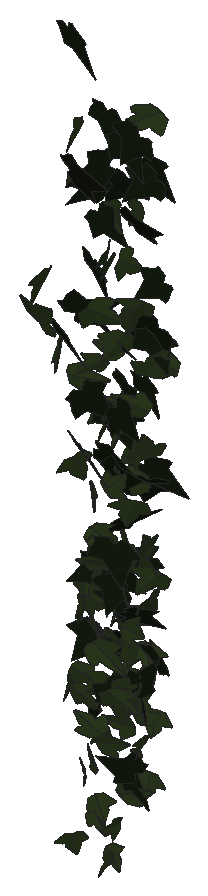
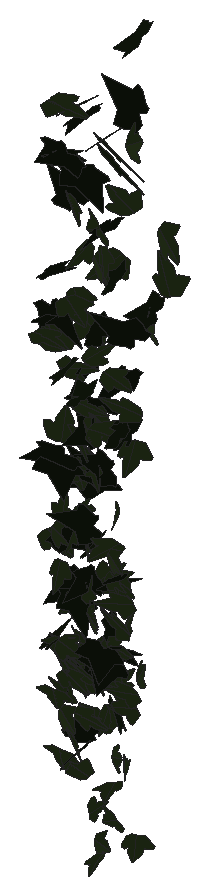
# SketchUp Ruby script. Lengths in inches.
U = 1.inch
M = Sketchup.active_model
def pt(a) = Geom::Point3d.new(a.map { |v| v * U })
def face(e, loops, mat)
  f = e.add_face(loops[0].map { |a| pt(a) })
  loops[1..].each { |l| e.add_face(l.map { |a| pt(a) }).erase! }
  f.material = f.back_material = mat if mat
  f
end
# faces: each face lists its corners as indices into pts; further lists are holes
def faces(e, pts, list, mat = nil) = list.each { |f| face(e, (f[0].is_a?(Array) ? f : [f]).map { |l| l.map { |i| pts[i] } }, mat) }
# xy, xz, yz: faces in a plane at the given z, y or x. An outline is a flat list of corners, or four numbers for a rectangle; further outlines are holes
def ring(l) = l.size == 4 ? [[l[0], l[1]], [l[2], l[1]], [l[2], l[3]], [l[0], l[3]]] : l.each_slice(2).to_a
def flat(e, list, mat, &to3) = list.each { |f| face(e, (f[0].is_a?(Array) ? f : [f]).map { |l| ring(l).map { |u, v| to3.(u, v) } }, mat) }
def xy(e, z, list, mat = nil) = flat(e, list, mat) { |x, y| [x, y, z] }
def xz(e, y, list, mat = nil) = flat(e, list, mat) { |x, z| [x, y, z] }
def yz(e, x, list, mat = nil) = flat(e, list, mat) { |y, z| [x, y, z] }
def lines(e, pts, list) = list.each { |a, b| e.add_line(pt(pts[a]), pt(pts[b])) }
# prism: a flat outline (further loops are holes) pulled along v
def prism(e, loops, v, mat = nil)
  f = face(e, loops, mat); d = Geom::Vector3d.new(v.map { |x| x * U })
  f.pushpull(f.normal.samedirection?(d) ? d.length : -d.length)
end
def box(e, o, s, mat = nil) = prism(e, [[o, [o[0] + s[0], o[1], o[2]], [o[0] + s[0], o[1] + s[1], o[2]], [o[0], o[1] + s[1], o[2]]]], [0, 0, s[2]], mat)
def at(x, y, z, deg = 0) = Geom::Transformation.translation(pt([x, y, z])) * Geom::Transformation.rotation(ORIGIN, Z_AXIS, deg.degrees)
def axes(o, x, y, z) = Geom::Transformation.new([*x, 0, *y, 0, *z, 0, *pt(o).to_a, 1])
def part(name) = M.definitions.add(name)
# library, detail: a bought-in or finely detailed component or shape, given as its bounding box
def library(name, o, s) = part(name).tap { |d| box(d.entities, o, s) }
def detail(e, o, s) = box(e.add_group.entities, o, s)
def put(e, d, t, mat = nil) = e.add_instance(d, t).tap { |i| i.material = mat if mat }
def group(e, t, mat = nil) = e.add_group.tap { |g| g.transformation = t; g.material = mat if mat }.entities
root = M.entities
M.materials.add("1026 AP 7946 SUNNY SIDE UP").color = [254, 231, 186]
M.materials.add("efeu1").color = [18, 25, 13]
M.materials.add("efeu2").color = [43, 57, 29]
c1 = part("ivyleaf_10")
p = [[0,0.5,-0.03],[-0.0625,2.02,-0.43],[-0.19,2.01,-0.46],[-0.54,1.05,-0.29],[-0.52,0.625,-0.18],[-0.83,0.76,-0.28],
  [-1.16,0.64,-0.33],[-1.15,0.33,-0.24],[-0.77,-0.39,0.02],[-0.3,-0.51,0.16],[0.04,-0.48,0.23],[-0.02,2.01,-0.4375],
  [-0.06,2.01,-0.43],[0.04,-0.49,0.23],[0.67,-0.49,0.14],[1.38,0.36,-0.2],[1.375,0.51,-0.24],[0.81,0.65,-0.19],
  [0.62,0.59,-0.15],[0.6,1.09,-0.28],[0.5,1.23,-0.31]]
faces(c1.entities,p,[[0,1,2,3,4,5,6,7,8,9,10],[11,12,0,13,14,15,16,17,18,19,20]],"efeu2")
c2 = part("ivyleaf_9")
p = [[1.54,2.16,1.25],[1.36,2.04,1.19],[-0.21,0.99,0.68],[-0.71,1.11,0.82],[-0.85,0.86,0.67],[-0.8,0.17,0.21],
  [-0.9,-0.01,0.1],[-0.67,-0.16,-0.02],[-0.08,-0.08,-0.05],[-0.03,-0.6,-0.4],[0.65,-0.88,-0.66],[0.83,-0.6,-0.49],
  [1.29,-0.42,-0.43],[1.8125,-0.07,-0.26],[1.21,0.44,0.15]]
faces(c2.entities,p,[[0,1,2,3,4,5,6,7,8,9,10,11,12,13,14]],"efeu1")
put(root,c1,axes([106.32,210.03,262.625],[0.08292,-0.31995,0.11678],[0.03412,-0.11315,-0.33471],[0.5336,0.05695,0.00326]),"1026 AP 7946 SUNNY SIDE UP")
put(root,c2,axes([107.03,210.0625,265.32],[0.36461,-0.08477,-0.26189],[0.41394,0.01257,0.24359],[-0.07483,-0.3435,0.07141]),"1026 AP 7946 SUNNY SIDE UP")
put(root,c1,axes([106.15,210.07,261.48],[-0.42812,0.06677,0.19799],[0.28105,-0.07357,0.28733],[0.15166,0.32482,0.02646]),"1026 AP 7946 SUNNY SIDE UP")
put(root,c1,axes([107.52,210.3125,254.02],[0.2513,0.07628,0.2158],[0.32134,0.05151,-0.18003],[-0.13844,0.25804,-0.02615]),"1026 AP 7946 SUNNY SIDE UP")
put(root,c1,axes([106.29,210.54,260.7],[0.12846,-0.09926,0.28623],[0.25636,-0.22579,-0.13354],[0.38765,0.18221,-0.00653]),"1026 AP 7946 SUNNY SIDE UP")
put(root,c2,axes([107.8,210.52,256.46],[-0.16884,-0.23575,-0.10816],[0.09206,0.08701,-0.26586],[0.39433,-0.12125,0.01575]),"1026 AP 7946 SUNNY SIDE UP")
put(root,c1,axes([107.26,210.54,251.91],[0.14816,0.17283,0.13537],[-0.1153,-0.10836,0.20187],[0.32033,-0.11894,0.01005]),"1026 AP 7946 SUNNY SIDE UP")
put(root,c2,axes([106.14,210.61,261.12],[0.282,-0.2341,0.08241],[0.05534,-0.07531,-0.30373],[0.38573,0.18195,-0.01667]),"1026 AP 7946 SUNNY SIDE UP")
put(root,c1,axes([107.27,210.46,261.93],[-0.17759,-0.15909,-0.25489],[0.26554,0.18076,-0.19882],[0.37724,-0.20212,0.01995]),"1026 AP 7946 SUNNY SIDE UP")
put(root,c1,axes([106.34,210.83,252.49],[0.01742,0.01744,0.23633],[0.18302,-0.19843,0.00859],[0.31187,0.11547,-0.01824]),"1026 AP 7946 SUNNY SIDE UP")
put(root,c2,axes([106.57,210.89,258.23],[0.2136,-0.22227,0.16698],[0.10655,-0.14961,-0.26866],[0.42044,0.15084,-0.01675]),"1026 AP 7946 SUNNY SIDE UP")
put(root,c1,axes([107.51,210.83,252.68],[-0.27027,-0.05091,-0.17004],[0.26003,0.01732,-0.18313],[0.0769,-0.23747,0.02163]),"1026 AP 7946 SUNNY SIDE UP")
put(root,c1,axes([107.79,211.07,255.99],[-0.07859,-0.04134,0.25897],[0.06328,-0.25447,-0.03633],[0.39593,0.03246,0.05721]),"1026 AP 7946 SUNNY SIDE UP")
put(root,c2,axes([107.63,210.81,259.52],[0.14484,-0.18388,-0.23359],[-0.18555,0.19282,-0.21033],[0.41847,0.14915,-0.01241]),"1026 AP 7946 SUNNY SIDE UP")
put(root,c1,axes([106.47,210.87,257.91],[-0.16445,-0.25388,-0.116],[0.10257,0.09292,-0.28132],[0.42355,-0.12108,0.02309]),"1026 AP 7946 SUNNY SIDE UP")
put(root,c2,axes([107.12,210.98,264.7],[-0.41527,0.1572,-0.06447],[0.06317,-0.05612,-0.31572],[-0.25899,-0.26576,0.02637]),"1026 AP 7946 SUNNY SIDE UP")
put(root,c2,axes([106.125,211.11,267.87],[0.23929,-0.28624,0.02162],[-0.00227,-0.02636,-0.33383],[0.45148,0.15158,-0.01314]),"1026 AP 7946 SUNNY SIDE UP")
put(root,c2,axes([106.69,210.88,259.59],[0.06429,-0.13201,-0.28736],[-0.10817,0.26962,-0.14065],[0.47194,0.07978,0.00691]),"1026 AP 7946 SUNNY SIDE UP")
put(root,c2,axes([107.12,211.06,265.02],[-0.43631,0.14255,-0.03459],[0.02741,-0.041,-0.32029],[-0.22895,-0.27658,0.02757]),"1026 AP 7946 SUNNY SIDE UP")
put(root,c2,axes([107.76,211.15,250.78],[-0.02365,0.01928,0.25035],[-0.35632,-0.09056,-0.00758],[0.14083,-0.22589,0.02286]),"1026 AP 7946 SUNNY SIDE UP")
put(root,c1,axes([106.45,211.16,250.35],[-0.09375,0.04761,0.2054],[0.21823,-0.14305,0.07721],[0.23663,0.15078,0.01017]),"1026 AP 7946 SUNNY SIDE UP")
put(root,c1,axes([107.82,210.91,254.32],[0.01367,0.14138,0.19837],[-0.01664,0.19192,-0.14416],[-0.37423,-0.00337,0.01366]),"1026 AP 7946 SUNNY SIDE UP")
put(root,c1,axes([106.25,211.07,248.77],[-0.20399,-0.17666,-0.03485],[0.04792,0.01826,-0.22526],[0.27844,-0.13257,0.01324]),"1026 AP 7946 SUNNY SIDE UP")
put(root,c1,axes([107.01,211.08,251.26],[-0.18275,-0.01301,0.23093],[0.34586,0.04452,0.12037],[-0.0715,0.24861,-0.00797]),"1026 AP 7946 SUNNY SIDE UP")
put(root,c1,axes([107.8,211.125,257.17],[-0.28312,-0.18432,0.05319],[-0.03368,-0.05247,-0.26489],[0.29955,-0.18012,0.02049]),"1026 AP 7946 SUNNY SIDE UP")
put(root,c1,axes([107.1,211.24,248.49],[0.05113,-0.13791,0.15889],[0.05064,-0.15166,-0.14684],[0.3223,0.04571,-0.00214]),"1026 AP 7946 SUNNY SIDE UP")
put(root,c1,axes([106.88,211.08,249.85],[0.13379,0.20633,0.03103],[0.03031,0.02335,-0.22961],[-0.32621,0.0868,-0.00861]),"1026 AP 7946 SUNNY SIDE UP")
put(root,c1,axes([107.23,211.2,252.14],[-0.2718,0.02856,0.17064],[0.25305,-0.03965,0.18],[0.07541,0.23599,0.01103]),"1026 AP 7946 SUNNY SIDE UP")
put(root,c1,axes([107.15,211.15,257.36],[0.28593,-0.08077,-0.11673],[0.17478,-0.02659,0.20397],[-0.13064,-0.21236,0.01741]),"1026 AP 7946 SUNNY SIDE UP")
put(root,c1,axes([106.12,211.38,265.44],[0.0951,-0.07847,0.29999],[0.191,-0.266,-0.10124],[0.43479,0.13402,-0.02114]),"1026 AP 7946 SUNNY SIDE UP")
put(root,c1,axes([107.2,211.33,249.25],[-0.01882,-0.01293,-0.21646],[-0.09929,-0.20046,0.01525],[-0.31564,0.06383,0.00811]),"1026 AP 7946 SUNNY SIDE UP")
put(root,c2,axes([107.71,211.4,265.77],[-0.17456,-0.2176,0.16281],[-0.03602,-0.16401,-0.24825],[0.42248,-0.10389,0.0461]),"1026 AP 7946 SUNNY SIDE UP")
put(root,c1,axes([107.91,211.25,259.46],[0.09828,0.06504,0.22198],[-0.2881,-0.11453,0.08985],[0.2046,-0.19252,0.01989]),"1026 AP 7946 SUNNY SIDE UP")
put(root,c2,axes([107.46,211.25,265.68],[0.07827,-0.26682,-0.1117],[-0.03624,0.10445,-0.27899],[0.45053,0.05476,-0.00304]),"1026 AP 7946 SUNNY SIDE UP")
put(root,c1,axes([106.96,211.11,251.58],[-0.04173,-0.19174,-0.16902],[0.06072,0.15883,-0.19806],[0.391,-0.04513,0.01272]),"1026 AP 7946 SUNNY SIDE UP")
put(root,c1,axes([106.9,211.3125,252.64],[-0.17447,-0.11602,0.14727],[-0.12971,-0.11875,-0.16518],[0.25971,-0.13724,0.01644]),"1026 AP 7946 SUNNY SIDE UP")
put(root,c2,axes([107.09,211.41,254.93],[-0.11379,-0.23206,0.07154],[-0.02384,-0.06938,-0.25076],[0.38074,-0.0737,0.00568]),"1026 AP 7946 SUNNY SIDE UP")
put(root,c1,axes([106.2,211.42,254.03],[-0.03431,0.03747,0.2359],[0.17226,-0.20084,0.04348],[0.32125,0.1117,0.00188]),"1026 AP 7946 SUNNY SIDE UP")
put(root,c2,axes([106.77,211.11,251.76],[-0.14667,0.04437,-0.23639],[-0.30658,0.12194,0.10654],[0.20333,0.21587,-0.00987]),"1026 AP 7946 SUNNY SIDE UP")
put(root,c1,axes([106.74,211.15,250.61],[-0.08231,0.08241,-0.1968],[-0.13878,0.17011,0.10127],[0.29698,0.10233,-0.00722]),"1026 AP 7946 SUNNY SIDE UP")
put(root,c2,axes([107.22,211.1875,252.32],[-0.25833,-0.0618,0.17955],[0.23879,0.08876,0.18005],[-0.16683,0.22274,-0.02032]),"1026 AP 7946 SUNNY SIDE UP")
put(root,c2,axes([107.62,211.41,263.65],[0.00132,-0.10484,0.27286],[0.28123,-0.20668,-0.08588],[0.34973,0.16659,0.06803]),"1026 AP 7946 SUNNY SIDE UP")
put(root,c1,axes([107.27,211.4,260.84],[-0.19558,-0.2003,0.1471],[-0.05811,-0.14424,-0.24054],[0.38346,-0.12402,0.03858]),"1026 AP 7946 SUNNY SIDE UP")
put(root,c1,axes([107.67,211.24,252.39],[0.15047,-0.20183,-0.12557],[-0.09663,0.10436,-0.22929],[0.35696,0.11333,-0.00914]),"1026 AP 7946 SUNNY SIDE UP")
put(root,c1,axes([106.9,211.43,252.39],[0.04006,-0.00479,0.23746],[0.29797,-0.13169,-0.02517],[0.20653,0.19092,-0.00975]),"1026 AP 7946 SUNNY SIDE UP")
put(root,c2,axes([107.29,211.48,254.54],[0.02405,-0.22644,-0.09817],[0.0286,-0.09288,0.23299],[-0.38445,-0.02107,0.01119]),"1026 AP 7946 SUNNY SIDE UP")
put(root,c2,axes([107.09,211.52,255.59],[-0.0268,-0.18121,0.18577],[-0.02076,-0.1809,-0.18854],[0.40259,-0.02139,0.00264]),"1026 AP 7946 SUNNY SIDE UP")
put(root,c1,axes([108.19,211.41,255.48],[-0.24824,-0.13606,0.16015],[-0.14,-0.1328,-0.21261],[0.29414,-0.17804,0.03397]),"1026 AP 7946 SUNNY SIDE UP")
put(root,c1,axes([107.92,211.18,252.9],[0.01848,-0.06419,-0.21735],[-0.08294,0.20395,-0.06588],[0.33613,0.05385,-0.0043]),"1026 AP 7946 SUNNY SIDE UP")
put(root,c1,axes([107.92,211.45,256.07],[-0.03593,-0.20078,-0.13984],[-0.03914,-0.13252,0.20723],[-0.37806,0.0328,-0.00817]),"1026 AP 7946 SUNNY SIDE UP")
put(root,c1,axes([106.55,211.39,249.27],[0.19856,-0.01402,0.169],[0.25029,-0.04284,-0.13019],[0.06665,0.2026,-0.01459]),"1026 AP 7946 SUNNY SIDE UP")
put(root,c1,axes([106.16,211.375,252.07],[-0.1685,0.01707,-0.20591],[0.28924,-0.0823,-0.10927],[-0.12621,-0.21142,0.02448]),"1026 AP 7946 SUNNY SIDE UP")
put(root,c1,axes([107.34,211.23,252.61],[0.01536,0.00753,0.22374],[0.21383,0.1693,-0.01136],[-0.26644,0.13631,0.00378]),"1026 AP 7946 SUNNY SIDE UP")
put(root,c1,axes([107.19,211.45,258.79],[0.26508,-0.18734,0.09747],[0.07656,-0.08453,-0.25939],[0.32179,0.17444,-0.01858]),"1026 AP 7946 SUNNY SIDE UP")
put(root,c2,axes([107.52,211.38,250.57],[0.13643,-0.21638,-0.07815],[-0.05397,0.06661,-0.23968],[0.35584,0.09307,-0.00639]),"1026 AP 7946 SUNNY SIDE UP")
put(root,c2,axes([106.625,211.31,253.91],[0.30184,-0.09989,-0.14732],[-0.21809,0.04017,-0.22135],[0.16514,0.23564,-0.02305]),"1026 AP 7946 SUNNY SIDE UP")
put(root,c1,axes([107.46,211.32,250.07],[-0.17275,-0.04142,0.18244],[0.23487,0.09796,0.11949],[-0.16377,0.18417,-0.02108]),"1026 AP 7946 SUNNY SIDE UP")
put(root,c1,axes([106.39,211.43,254.92],[0.3209,-0.05476,0.06617],[0.08855,-0.03792,-0.21682],[0.09936,0.21066,-0.02047]),"1026 AP 7946 SUNNY SIDE UP")
put(root,c2,axes([107.9,211.29,252.47],[0.15152,-0.06702,-0.22121],[-0.31781,0.07581,-0.11758],[0.15396,0.22245,-0.02501]),"1026 AP 7946 SUNNY SIDE UP")
put(root,c2,axes([107.59,211.23,254.48],[0.33258,0.13179,0.09379],[0.13358,0.03408,-0.25607],[-0.21273,0.22744,-0.01416]),"1026 AP 7946 SUNNY SIDE UP")
put(root,c1,axes([106.84,211.54,258.75],[0.11008,-0.19133,0.18866],[0.08502,-0.17625,-0.21078],[0.40888,0.08816,-0.00696]),"1026 AP 7946 SUNNY SIDE UP")
put(root,c2,axes([107.12,211.43,259.07],[-0.1834,-0.17381,-0.17685],[0.17773,0.12902,-0.21417],[0.33931,-0.16152,0.01659]),"1026 AP 7946 SUNNY SIDE UP")
put(root,c2,axes([106.82,211.52,260.75],[0.14781,-0.15862,0.1983],[0.1804,-0.15623,-0.19038],[0.34947,0.14774,0.01441]),"1026 AP 7946 SUNNY SIDE UP")
put(root,c2,axes([106.55,211.64,254.99],[-0.20291,-0.12232,0.19602],[-0.18709,-0.15053,-0.18304],[0.30357,-0.17453,0.01821]),"1026 AP 7946 SUNNY SIDE UP")
put(root,c2,axes([106.36,211.6,262.24],[0.11963,-0.22475,0.14172],[0.04055,-0.13748,-0.24463],[0.41342,0.07852,-0.01702]),"1026 AP 7946 SUNNY SIDE UP")
put(root,c1,axes([106.67,211.58,255.12],[-0.10183,-0.07017,-0.20896],[-0.18161,-0.16669,0.09661],[-0.28375,0.13187,0.01315]),"1026 AP 7946 SUNNY SIDE UP")
put(root,c2,axes([107.76,211.58,255.7],[0.00761,-0.01345,-0.26186],[-0.09683,-0.24666,0.0108],[-0.38823,0.06126,-0.00783]),"1026 AP 7946 SUNNY SIDE UP")
put(root,c1,axes([106.07,211.47,252.48],[-0.11802,-0.02078,-0.21997],[0.32536,-0.06629,-0.06871],[-0.08838,-0.21629,0.0408]),"1026 AP 7946 SUNNY SIDE UP")
put(root,c2,axes([107.73,211.35,252.67],[-0.21899,0.20479,0.09455],[0.09835,-0.06689,0.25438],[0.33811,0.15209,-0.01275]),"1026 AP 7946 SUNNY SIDE UP")
put(root,c1,axes([107.78,211.53,251.42],[0.04289,-0.22308,0.0796],[0.00767,-0.07851,-0.23194],[0.3718,0.02735,-0.0044]),"1026 AP 7946 SUNNY SIDE UP")
put(root,c1,axes([106.44,211.54,255.16],[-0.13008,-0.16277,0.12732],[-0.07179,-0.11627,-0.18851],[0.31415,-0.09397,0.00964]),"1026 AP 7946 SUNNY SIDE UP")
put(root,c2,axes([106.95,211.55,257.38],[0.04042,-0.0091,0.26543],[0.24809,-0.20428,-0.02484],[0.3207,0.15918,-0.01424]),"1026 AP 7946 SUNNY SIDE UP")
put(root,c2,axes([106.48,211.61,253.46],[-0.34908,-0.13128,0.01188],[0.00299,-0.02723,-0.26467],[0.20731,-0.22067,0.02382]),"1026 AP 7946 SUNNY SIDE UP")
put(root,c2,axes([107.92,211.65,264.72],[-0.27669,-0.14947,0.09921],[-0.09524,-0.07827,-0.23751],[0.26364,-0.18514,0.01833]),"1026 AP 7946 SUNNY SIDE UP")
put(root,c1,axes([107.8,211.44,255.75],[-0.35025,0.12442,0.03747],[-0.06596,-0.00224,-0.26186],[-0.19253,-0.22557,0.02155]),"1026 AP 7946 SUNNY SIDE UP")
put(root,c1,axes([106.84,211.5625,262.46],[0.11156,-0.26195,0.05664],[0.00662,-0.05731,-0.27971],[0.42131,0.07027,-0.0106]),"1026 AP 7946 SUNNY SIDE UP")
put(root,c1,axes([107.47,211.52,261.47],[-0.12674,-0.26375,-0.00845],[0.01643,0.00381,-0.28395],[0.41453,-0.08079,0.00868]),"1026 AP 7946 SUNNY SIDE UP")
put(root,c1,axes([106.49,211.62,259.93],[-0.12988,-0.12168,0.17534],[-0.12468,-0.15193,-0.15182],[0.3054,-0.11377,0.01259]),"1026 AP 7946 SUNNY SIDE UP")
put(root,c1,axes([107.625,211.49,250.94],[0.17154,-0.18297,-0.09149],[-0.09004,0.06784,-0.21863],[0.30612,0.12248,-0.01304]),"1026 AP 7946 SUNNY SIDE UP")
put(root,c1,axes([107.58,211.64,257.4],[-0.06391,0.01487,0.24591],[-0.24806,-0.18354,-0.01698],[0.28247,-0.15781,0.04073]),"1026 AP 7946 SUNNY SIDE UP")
put(root,c1,axes([107.83,211.57,250.52],[0.35393,-0.00733,0.02512],[0.03727,-0.01988,-0.2313],[0.01479,0.22554,-0.01825]),"1026 AP 7946 SUNNY SIDE UP")
put(root,c2,axes([107,211.53,252.97],[-0.01724,-0.21196,0.15463],[0.02944,0.1504,0.21934],[-0.40843,0.01979,0.00928]),"1026 AP 7946 SUNNY SIDE UP")
put(root,c1,axes([107.42,211.4375,254.3],[-0.13108,-0.13426,-0.1951],[0.18553,0.14784,-0.16128],[0.31322,-0.14376,0.01388]),"1026 AP 7946 SUNNY SIDE UP")
put(root,c1,axes([107.75,211.66,258.14],[-0.22471,-0.22236,-0.09819],[-0.07631,-0.0806,0.27182],[-0.37187,0.1509,0.00355]),"1026 AP 7946 SUNNY SIDE UP")
put(root,c1,axes([107.95,211.47,254.83],[-0.07024,-0.21746,-0.15541],[0.03957,0.14755,-0.2278],[0.41317,-0.0511,-0.0046]),"1026 AP 7946 SUNNY SIDE UP")
put(root,c1,axes([107.77,211.51,251.92],[0.33714,-0.04967,0.09346],[-0.13084,0.04223,0.22598],[-0.09722,-0.22906,0.01995]),"1026 AP 7946 SUNNY SIDE UP")
put(root,c1,axes([107.52,211.54,258.22],[0.26762,-0.18113,-0.12956],[-0.13929,0.0879,-0.2555],[0.31651,0.19183,-0.0029]),"1026 AP 7946 SUNNY SIDE UP")
put(root,c1,axes([107.39,211.57,253.48],[0.25254,-0.16292,-0.06673],[-0.08132,0.03861,-0.23526],[0.26286,0.16847,-0.00866]),"1026 AP 7946 SUNNY SIDE UP")
put(root,c1,axes([106.78,211.5,262.7],[0.04104,-0.24552,-0.13626],[-0.02356,0.13002,-0.25359],[0.43684,0.03008,-0.00088]),"1026 AP 7946 SUNNY SIDE UP")
put(root,c1,axes([107.3,211.54,251.57],[0.05116,-0.02135,-0.23197],[-0.33047,0.08087,-0.03873],[0.1309,0.21252,-0.00713]),"1026 AP 7946 SUNNY SIDE UP")
put(root,c1,axes([107.82,211.71,255.84],[0.01324,-0.19134,0.14574],[0.01019,-0.14241,-0.19814],[0.37505,0.01062,0.00024]),"1026 AP 7946 SUNNY SIDE UP")
put(root,c1,axes([106.09,211.52,264.0625],[-0.17307,-0.20334,0.14503],[0.09637,0.12816,0.23887],[-0.37783,0.12583,-0.00551]),"1026 AP 7946 SUNNY SIDE UP")
put(root,c2,axes([106.01,211.51,260.97],[-0.02616,0.02137,0.27757],[0.4234,-0.02056,0.0187],[0.03443,0.26904,-0.01903]),"1026 AP 7946 SUNNY SIDE UP")
put(root,c1,axes([107.23,211.52,255.93],[0.11644,-0.18688,-0.13933],[-0.05099,0.13108,-0.20573],[0.35814,0.07942,0.01601]),"1026 AP 7946 SUNNY SIDE UP")
put(root,c1,axes([107.92,211.58,260.2],[-0.30487,-0.19343,0.0784],[0.06209,0.06942,0.28176],[-0.32153,0.1968,-0.01993]),"1026 AP 7946 SUNNY SIDE UP")
put(root,c1,axes([107.25,211.46,262.64],[0.00822,-0.17777,-0.22482],[0.17545,0.20067,-0.16524],[0.40498,-0.08333,0.07615]),"1026 AP 7946 SUNNY SIDE UP")
put(root,c1,axes([106.15,211.55,254.62],[-0.09457,-0.03504,-0.22856],[0.34498,0.03908,-0.06746],[0.07421,-0.22633,0.02234]),"1026 AP 7946 SUNNY SIDE UP")
put(root,c2,axes([107.25,211.6,264.52],[0.20087,0.1064,-0.23073],[-0.23077,-0.17146,-0.1707],[-0.31532,0.19327,-0.02205]),"1026 AP 7946 SUNNY SIDE UP")
put(root,c2,axes([106.58,211.55,263.49],[0.13708,-0.19077,-0.19265],[-0.07169,0.18205,-0.2134],[0.41268,0.09499,0.02692]),"1026 AP 7946 SUNNY SIDE UP")
put(root,c1,axes([106.89,211.74,260.28],[0.02071,0.15154,0.21575],[-0.06404,-0.20499,0.15489],[0.40029,-0.04064,0.01362]),"1026 AP 7946 SUNNY SIDE UP")
put(root,c1,axes([106.25,211.7,256.79],[-0.0843,0.16409,-0.15328],[0.05902,-0.14512,-0.17854],[-0.34426,-0.06506,0.00693]),"1026 AP 7946 SUNNY SIDE UP")
put(root,c2,axes([107.46,211.53,254.31],[0.02401,0.2524,-0.06237],[-0.00358,-0.06195,-0.26086],[-0.40865,0.01538,-0.00138]),"1026 AP 7946 SUNNY SIDE UP")
put(root,c1,axes([106.99,211.54,257.56],[-0.23975,0.10167,0.13426],[-0.18762,0.05387,-0.18762],[-0.17883,-0.19282,0.01685]),"1026 AP 7946 SUNNY SIDE UP")
put(root,c1,axes([107.15,211.62,254.58],[-0.2989,0.19808,0.01203],[0.02954,0.00343,0.28237],[0.3105,0.19035,-0.01529]),"1026 AP 7946 SUNNY SIDE UP")
put(root,c2,axes([106.51,211.67,257.75],[0.14025,-0.01329,-0.24906],[0.37223,0.05851,0.08703],[0.07939,-0.25089,0.03194]),"1026 AP 7946 SUNNY SIDE UP")
put(root,c1,axes([106.0625,211.74,254.12],[0.04004,-0.07107,-0.26468],[0.32042,-0.16058,0.06573],[-0.26927,-0.20165,0.03886]),"1026 AP 7946 SUNNY SIDE UP")
put(root,c1,axes([107.92,211.68,251.97],[0.34717,0.01388,0.01006],[0.01725,-0.02085,-0.22695],[-0.02027,0.22002,-0.02083]),"1026 AP 7946 SUNNY SIDE UP")
put(root,c1,axes([106.34,211.74,255.72],[0.07497,-0.20027,0.08404],[0.02082,-0.08185,-0.21248],[0.34008,0.04916,-0.00552]),"1026 AP 7946 SUNNY SIDE UP")
put(root,c1,axes([106.45,211.5625,253.49],[-0.05768,0.00373,-0.23322],[-0.28094,0.14043,0.03303],[0.21874,0.18134,-0.01908]),"1026 AP 7946 SUNNY SIDE UP")
put(root,c1,axes([107.56,211.6875,252.5],[-0.21559,-0.02457,0.16654],[-0.23232,-0.07217,-0.1407],[0.11065,-0.19942,0.02907]),"1026 AP 7946 SUNNY SIDE UP")
put(root,c1,axes([106.82,211.59,248.39],[0.01186,0.21824,0.06228],[0.0062,0.05911,-0.22461],[-0.35551,0.00831,-0.00184]),"1026 AP 7946 SUNNY SIDE UP")
put(root,c1,axes([107.07,211.69,252.625],[0.14697,-0.09948,-0.20095],[0.30388,-0.06098,0.12745],[-0.16016,-0.20699,0.05743]),"1026 AP 7946 SUNNY SIDE UP")
put(root,c1,axes([106.83,211.7,253.15],[-0.366,-0.06512,-0.06547],[-0.10316,0.00065,0.24833],[-0.09855,0.24118,-0.01683]),"1026 AP 7946 SUNNY SIDE UP")
put(root,c1,axes([106.48,211.55,255.87],[0.14929,0.15349,0.19104],[0.15474,0.15615,-0.18501],[-0.34428,0.13674,-0.00032]),"1026 AP 7946 SUNNY SIDE UP")
put(root,c2,axes([107.54,211.77,259.77],[0.13562,-0.23927,0.02279],[0.00005,-0.02493,-0.26202],[0.37804,0.08584,-0.00814]),"1026 AP 7946 SUNNY SIDE UP")
put(root,c2,axes([107.84,211.75,260.9375],[-0.06765,-0.2357,-0.10701],[0.07316,0.0951,-0.24478],[0.39749,-0.05762,0.02684]),"1026 AP 7946 SUNNY SIDE UP")
put(root,c1,axes([105.86,211.67,259.33],[0.07658,-0.02948,-0.26044],[0.39928,-0.00924,0.05149],[-0.02314,-0.25713,0.02648]),"1026 AP 7946 SUNNY SIDE UP")
put(root,c1,axes([107.75,211.75,252.9],[0.25144,-0.15985,0.01707],[0.00212,-0.02331,-0.23252],[0.25284,0.15916,-0.01503]),"1026 AP 7946 SUNNY SIDE UP")
put(root,c2,axes([106.09,211.84,258.71],[0.10663,-0.17354,0.16601],[0.10971,-0.14661,-0.19259],[0.35696,0.0969,0.0096]),"1026 AP 7946 SUNNY SIDE UP")
put(root,c1,axes([107.23,211.74,259.07],[-0.0456,0.06309,0.22267],[-0.33121,-0.08369,-0.00444],[0.12358,-0.201,0.07025]),"1026 AP 7946 SUNNY SIDE UP")
put(root,c2,axes([106.54,211.63,253.17],[0.32052,0.1363,-0.07746],[-0.07926,-0.06075,-0.252],[-0.2322,0.20888,-0.0209]),"1026 AP 7946 SUNNY SIDE UP")
put(root,c1,axes([106.83,211.84,254.2],[0.14351,-0.16618,0.14745],[0.10585,-0.1274,-0.19606],[0.32924,0.11339,-0.00124]),"1026 AP 7946 SUNNY SIDE UP")
put(root,c1,axes([107.46,211.71,263.83],[0.2536,-0.17153,-0.07523],[-0.06218,0.06157,-0.24184],[0.28586,0.16557,0.01413]),"1026 AP 7946 SUNNY SIDE UP")
put(root,c2,axes([106.97,211.5625,255.02],[0.00501,-0.0506,-0.2778],[-0.07385,0.2653,-0.05036],[0.42459,0.04674,-0.00548]),"1026 AP 7946 SUNNY SIDE UP")
put(root,c1,axes([107.51,211.875,253.33],[-0.08134,-0.16334,0.17996],[-0.03455,-0.17567,-0.17602],[0.37554,-0.05154,0.02279]),"1026 AP 7946 SUNNY SIDE UP")
put(root,c2,axes([107.01,211.94,259.375],[-0.02638,-0.18393,0.19711],[0.06766,-0.1921,-0.18646],[0.41299,0.01972,0.04314]),"1026 AP 7946 SUNNY SIDE UP")
put(root,c2,axes([107.92,211.88,253.21],[0.10896,-0.2341,-0.02031],[0.01915,-0.01556,0.25131],[-0.36873,-0.06998,0.00705]),"1026 AP 7946 SUNNY SIDE UP")
put(root,c1,axes([107.73,211.86,266.1],[0.23274,0.08233,-0.23859],[-0.30805,-0.12465,-0.17502],[-0.23456,0.24541,-0.00689]),"1026 AP 7946 SUNNY SIDE UP")
put(root,c2,axes([107.77,211.69,257.49],[0.21654,0.17571,-0.12845],[-0.10579,-0.10675,-0.23032],[-0.3228,0.15286,-0.01068]),"1026 AP 7946 SUNNY SIDE UP")
put(root,c2,axes([106.82,211.76,258.59],[0.35699,-0.09948,0.01162],[0.0047,-0.02261,-0.2547],[0.15745,0.22621,-0.01875]),"1026 AP 7946 SUNNY SIDE UP")
put(root,c1,axes([106.6,211.95,258.72],[-0.12954,-0.09783,0.24392],[-0.06913,-0.24019,-0.11913],[0.39767,-0.07362,0.05875]),"1026 AP 7946 SUNNY SIDE UP")
put(root,c1,axes([108.13,211.84,260.46],[0.24468,0.03173,-0.17441],[-0.24823,-0.06558,-0.16236],[-0.10902,0.22053,-0.02176]),"1026 AP 7946 SUNNY SIDE UP")
put(root,c2,axes([107.92,211.76,261.13],[0.12207,0.00774,-0.28097],[-0.39288,-0.11201,-0.07719],[-0.17253,0.26056,-0.02303]),"1026 AP 7946 SUNNY SIDE UP")
put(root,c2,axes([107.53,211.8,264.95],[-0.10526,-0.05873,-0.28037],[0.38002,0.12602,-0.08863],[0.21631,-0.24997,0.01927]),"1026 AP 7946 SUNNY SIDE UP")
put(root,c1,axes([106.9,211.87,258.71],[0.13262,-0.19395,0.07857],[0.04668,-0.07146,-0.21829],[0.325,0.08941,-0.00071]),"1026 AP 7946 SUNNY SIDE UP")
put(root,c2,axes([106.45,211.94,265.69],[-0.00617,-0.25496,0.05987],[0.01035,-0.05964,-0.26293],[0.41156,-0.00232,0.00751]),"1026 AP 7946 SUNNY SIDE UP")
put(root,c1,axes([106.56,211.9,263.52],[0.22203,-0.051,0.241],[0.32951,-0.10573,-0.15449],[0.18302,0.25223,-0.01423]),"1026 AP 7946 SUNNY SIDE UP")
put(root,c2,axes([107.86,211.99,262.1],[-0.17871,-0.14659,0.16576],[-0.13931,-0.13568,-0.19161],[0.31368,-0.14376,0.00934]),"1026 AP 7946 SUNNY SIDE UP")
put(root,c2,axes([107.05,211.62,254.45],[0.0015,0.02617,0.26569],[0.00274,0.25775,-0.02546],[-0.40736,0.00183,0.00081]),"1026 AP 7946 SUNNY SIDE UP")
put(root,c1,axes([107.38,211.86,261.46],[-0.26298,-0.14107,0.12114],[-0.12358,-0.08996,-0.22533],[0.26189,-0.18411,0.01531]),"1026 AP 7946 SUNNY SIDE UP")
put(root,c2,axes([106.6,211.72,253.45],[0.25159,0.16087,-0.08512],[-0.07961,-0.06732,-0.23387],[-0.27368,0.16747,-0.01021]),"1026 AP 7946 SUNNY SIDE UP")
put(root,c1,axes([107.6,211.8,253.36],[0.24696,0.16239,0.02262],[0.04005,0.00457,-0.23219],[-0.25434,0.1584,-0.0146]),"1026 AP 7946 SUNNY SIDE UP")
put(root,c2,axes([107,211.62,256.23],[0.05219,0.23332,-0.14492],[0.02522,0.14113,0.24358],[0.42873,-0.0367,0.00331]),"1026 AP 7946 SUNNY SIDE UP")
put(root,c2,axes([107.625,211.78,257.76],[0.03814,-0.09971,-0.26037],[0.2797,0.19694,-0.06144],[0.32182,-0.15935,0.08426]),"1026 AP 7946 SUNNY SIDE UP")
